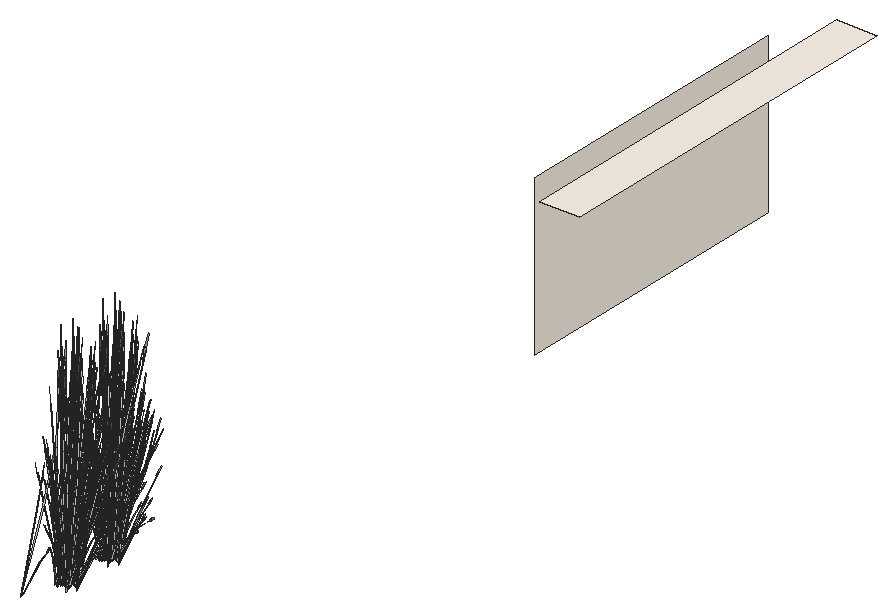
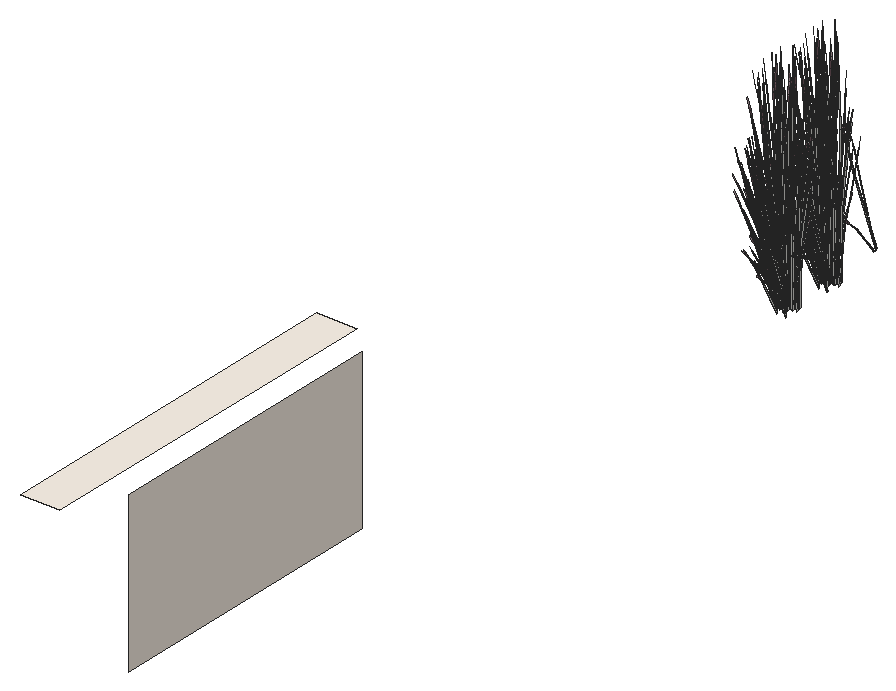
# SketchUp Ruby script. Lengths in inches.
U = 1.inch
M = Sketchup.active_model
def pt(a) = Geom::Point3d.new(a.map { |v| v * U })
def face(e, loops, mat)
  f = e.add_face(loops[0].map { |a| pt(a) })
  loops[1..].each { |l| e.add_face(l.map { |a| pt(a) }).erase! }
  f.material = f.back_material = mat if mat
  f
end
# faces: each face lists its corners as indices into pts; further lists are holes
def faces(e, pts, list, mat = nil) = list.each { |f| face(e, (f[0].is_a?(Array) ? f : [f]).map { |l| l.map { |i| pts[i] } }, mat) }
# xy, xz, yz: faces in a plane at the given z, y or x. An outline is a flat list of corners, or four numbers for a rectangle; further outlines are holes
def ring(l) = l.size == 4 ? [[l[0], l[1]], [l[2], l[1]], [l[2], l[3]], [l[0], l[3]]] : l.each_slice(2).to_a
def flat(e, list, mat, &to3) = list.each { |f| face(e, (f[0].is_a?(Array) ? f : [f]).map { |l| ring(l).map { |u, v| to3.(u, v) } }, mat) }
def xy(e, z, list, mat = nil) = flat(e, list, mat) { |x, y| [x, y, z] }
def xz(e, y, list, mat = nil) = flat(e, list, mat) { |x, z| [x, y, z] }
def yz(e, x, list, mat = nil) = flat(e, list, mat) { |y, z| [x, y, z] }
def lines(e, pts, list) = list.each { |a, b| e.add_line(pt(pts[a]), pt(pts[b])) }
# prism: a flat outline (further loops are holes) pulled along v
def prism(e, loops, v, mat = nil)
  f = face(e, loops, mat); d = Geom::Vector3d.new(v.map { |x| x * U })
  f.pushpull(f.normal.samedirection?(d) ? d.length : -d.length)
end
def box(e, o, s, mat = nil) = prism(e, [[o, [o[0] + s[0], o[1], o[2]], [o[0] + s[0], o[1] + s[1], o[2]], [o[0], o[1] + s[1], o[2]]]], [0, 0, s[2]], mat)
def at(x, y, z, deg = 0) = Geom::Transformation.translation(pt([x, y, z])) * Geom::Transformation.rotation(ORIGIN, Z_AXIS, deg.degrees)
def axes(o, x, y, z) = Geom::Transformation.new([*x, 0, *y, 0, *z, 0, *pt(o).to_a, 1])
def part(name) = M.definitions.add(name)
# library, detail: a bought-in or finely detailed component or shape, given as its bounding box
def library(name, o, s) = part(name).tap { |d| box(d.entities, o, s) }
def detail(e, o, s) = box(e.add_group.entities, o, s)
def put(e, d, t, mat = nil) = e.add_instance(d, t).tap { |i| i.material = mat if mat }
def group(e, t, mat = nil) = e.add_group.tap { |g| g.transformation = t; g.material = mat if mat }.entities
root = M.entities
M.materials.add("C01_Vanilla_Cream").color = [255, 246, 235]
M.materials.add("LightPink_Translucent").color = [144, 107, 117]
M.materials["LightPink_Translucent"].alpha = 0.75
c1 = part("blade")
p = [[2.15,0.21,22],[0,0.17,0],[0.09,0.45,0],[2.18,0.31,22],[2.29,0.31,22],[0.38,0.45,0],
  [2.48,0.24,33],[2.49,0.24,33],[2.48,0.22,33]]
faces(c1.entities,p,[[0,1,2,3],[4,5,2,3],[6,3,4,7],[8,0,3,6]])
c2 = part("seeds")
p = [[0.3,-0.1,1.38],[-0.01,-0.03,1.59],[-0.01,-0.03,0.03],[0.14,-0.07,-0.07],[0.29,-0.03,3],[0.15,0.01,3.11]]
faces(c2.entities,p,[[0,1,2,3],[1,0,4,5]],"LightPink_Translucent")
c3 = part("blade with seeds")
put(c3.entities,c1,at(0,0,0))
put(c3.entities,c2,axes([2.4,0.25,30.99],[1.5799,-0.05474,1.17369],[-0.12525,1.92788,0.29478],[-0.07173,-0.02425,1.56792]))
xy(root,690,[[360,288,369,372]],"C01_Vanilla_Cream")
yz(root,354,[[294,654,360,690]],"C01_Vanilla_Cream")
put(root,c3,axes([341.72,163.8,657.71],[-0.14896,0.31857,-0.29039],[-0.4346,-0.09292,0.3749],[0.03985,0.12826,0.71734]))
put(root,c3,axes([341.77,163.52,658.08],[0.23583,0.33684,-0.58257],[-0.48546,0.18772,0.0703],[0.05515,0.16275,0.8241]))
put(root,c3,axes([341.41,164.37,657.87],[0.06263,0.06671,1.43454],[0.50546,0.02621,-0.22687],[0.05083,0.14712,0.11505]))
put(root,c3,axes([343.01,173.53,656.125],[-0.14045,0.08385,1.17261],[-0.42064,-0.14676,-0.25218],[0.07797,-0.18252,0.50135]))
put(root,c3,axes([343.35,174.15,658.08],[0.01286,-0.38319,-0.58257],[0.54141,0.02574,0.0703],[0.05714,-0.16234,0.8241]))
put(root,c3,axes([344.11,173.55,657.87],[-0.00477,-0.08245,1.43454],[-0.40285,-0.23829,-0.22687],[0.06228,-0.14445,0.11505]))
put(root,c3,axes([342.41,173.54,657.71],[0.14896,-0.31857,-0.29039],[0.4346,0.09292,0.3749],[-0.03985,-0.12826,0.71734]))
put(root,c3,axes([342.74,173.96,657.18],[-0.092,0.14239,1.40529],[-0.38596,-0.29467,0.11363],[0.17411,-0.18366,0.60075]))
put(root,c3,axes([344,173.26,657.86],[-0.05018,0.03164,1.45454],[-0.49165,-0.10676,-0.13744],[-0.0178,-0.13809,0.2574]))
put(root,c3,axes([342.49,172.86,656.27],[0.06339,0.24157,0.94186],[-0.35163,-0.13379,0.69201],[0.03784,-0.12369,0.20745]))
put(root,c3,axes([343.24,174.02,657.84],[-0.35372,-0.27835,-0.41901],[0.37366,-0.24377,-0.32456],[0.05382,-0.14142,0.80174]))
put(root,c3,axes([342.47,173.61,657.88],[0.48688,0.1083,0.39362],[-0.16649,0.35605,0.32456],[-0.02926,-0.14002,0.8145]))
put(root,c3,axes([343.61,174.17,658.13],[-0.54305,-0.02053,-0.09971],[0.01484,-0.38862,-0.55346],[0.03772,-0.14967,0.84097]))
put(root,c3,axes([343.57,173.92,657.71],[0.33433,-0.21811,-0.29039],[0.31649,0.24905,0.3749],[0.04815,-0.12654,0.71734]))
put(root,c3,axes([342.6,173.58,657.88],[0.36409,-0.14079,0.05273],[0.17821,0.25674,0.41509],[-0.03516,-0.11317,0.63295]))
put(root,c3,axes([343.99,173.79,655.22],[-0.07396,-0.03263,1.44601],[-0.18997,-0.3646,-0.2209],[0.12815,-0.09894,0.2463]))
put(root,c3,axes([343.57,174.01,657.88],[0.35185,0.28265,0.39362],[-0.37366,0.24377,0.32456],[0.0649,-0.13261,0.8145]))
put(root,c3,axes([343.7,174.03,657.88],[0.40605,0.0193,0.05273],[-0.01113,0.29147,0.41509],[0.04249,-0.11165,0.63295]))
put(root,c3,axes([343.4,174.23,658.14],[-0.33433,0.21811,0.29039],[-0.31649,-0.24905,-0.3749],[0.04815,-0.12654,0.71734]))
put(root,c3,axes([343.99,174.82,658.08],[0.2581,-0.32687,-0.58257],[0.45228,0.2323,0.0703],[0.15411,-0.11843,0.8241]))
put(root,c3,axes([341.2,173.87,655.95],[-0.30893,-0.41511,0],[0.51685,-0.2315,-0.42318],[0.11772,-0.05273,1.34243]))
put(root,c3,axes([343.98,174.67,657.84],[-0.12693,-0.37826,-0.41901],[0.48071,-0.06617,-0.32456],[0.13776,-0.1016,0.80174]))
put(root,c3,axes([344.2,174.9375,658.13],[-0.45707,-0.22842,-0.09971],[0.26332,-0.3308,-0.55346],[0.12913,-0.11499,0.84097]))
put(root,c3,axes([341.62,173.8,655.65],[0.46245,-0.20713,-0.40713],[0.27641,0.37142,0],[0.10533,-0.04718,1.29153]))
put(root,c3,axes([344.36,174.52,656.125],[-0.17652,-0.01227,1.17261],[-0.18084,-0.32916,-0.25218],[0.21685,-0.09312,0.50135]))
put(root,c3,axes([345.33,174.84,657.86],[-0.06454,-0.00315,1.45454],[-0.268,-0.33712,-0.13744],[0.10763,-0.11085,0.2574]))
put(root,c3,axes([342.17,174.65,655.6875],[0.33282,-0.31137,-0.51129],[0.41344,0.28235,-0.13419],[0.13336,-0.07767,1.12859]))
put(root,c3,axes([344.57,173.91,656.27],[-0.16458,0.21088,0.94186],[-0.14146,-0.28332,0.69201],[0.13593,-0.07099,0.20745]))
put(root,c3,axes([344.33,174.71,657.71],[0.43011,-0.0592,-0.29039],[0.11357,0.33844,0.3749],[0.12326,-0.0909,0.71734]))
put(root,c3,axes([341.59,175.2,655.8125],[0.23974,-0.37328,-0.36686],[0.49814,0.17965,0.17656],[0,-0.08605,1.17788]))
put(root,c3,axes([341.81,175.01,656.1875],[-0.05758,-0.4727,-0.23858],[0.59969,-0.02858,-0.41002],[0.1056,-0.06296,1.3096]))
put(root,c3,axes([343.98,174.91,658.14],[-0.43011,0.0592,0.29039],[-0.11357,-0.33844,-0.3749],[0.12326,-0.0909,0.71734]))
put(root,c3,axes([341.73,173.97,655.66],[0.46099,0.1025,-0.25402],[-0.11607,0.36097,0.25402],[0.09293,-0.04163,1.13959]))
put(root,c3,axes([344.37,174.85,657.88],[0.33921,0.17422,0.05273],[-0.19749,0.2481,0.41509],[0.10876,-0.08021,0.63295]))
put(root,c3,axes([344.27,174.78,657.88],[0.12254,0.38127,0.39362],[-0.48071,0.06617,0.32456],[0.14168,-0.08967,0.8145]))
put(root,c3,axes([345.57,175.24,657.87],[0.06857,-0.0631,1.43454],[-0.08776,-0.38707,-0.22687],[0.17204,-0.07339,0.11505]))
put(root,c3,axes([341.88,175.38,656],[0.55674,0.20078,0.19733],[-0.26794,0.4172,0.41002],[0,-0.09617,1.31645]))
put(root,c3,axes([341.7,175.1,656.23],[-0.53657,0.02557,0.36686],[-0.04852,-0.4245,-0.17656],[0.09606,-0.04302,1.17788]))
put(root,c3,axes([344.22,175.83,658.13],[-0.24861,-0.37512,-0.09971],[0.44125,-0.18434,-0.55346],[0.18594,-0.04949,0.84097]))
put(root,c3,axes([344.2,175.51,657.84],[0.13386,-0.37682,-0.41901],[0.45895,0.12916,-0.32456],[0.18478,-0.03455,0.80174]))
put(root,c3,axes([343.47,173.97,655.95],[0.30893,-0.41511,0],[0.51685,0.2315,-0.42318],[0.11772,0.05273,1.34243]))
put(root,c3,axes([341.69,175.26,655.9375],[0.21483,0.46323,0.37519],[-0.61383,0.16108,0.14723],[0.0075,-0.08512,1.30262]))
put(root,c3,axes([344.6875,175.61,655.625],[-0.31825,0.04971,1.16098],[-0.05066,-0.39572,0.06645],[0.2229,-0.0599,0.66064]))
put(root,c3,axes([345.27,175.26,655.85],[-0.30634,-0.2649,-0.0532],[0.33551,-0.24272,-0.24121],[0.09507,-0.01709,0.7956]))
put(root,c3,axes([342.46,175.3,655.81],[0,-0.47933,0],[0.61786,0,0],[0,0,1.47154]))
put(root,c3,axes([343.21,174.1875,656.03],[-0.46245,-0.20713,0.40713],[0.27641,-0.37142,0],[0.10533,0.04718,1.29153]))
put(root,c3,axes([344.11,175.64,658.08],[0.43419,-0.18296,-0.58257],[0.24197,0.37661,0.0703],[0.20979,-0.04278,0.8241]))
put(root,c3,axes([342.17,174.99,655.9375],[-0.40969,0.37595,0.37519],[-0.48673,-0.33186,0.14723],[0.09877,-0.03752,1.30262]))
put(root,c3,axes([341.45,174.375,656.03],[-0.14274,0.41171,0.14467],[-0.52234,-0.11651,0.28771],[0.09023,-0.00201,1.31534]))
put(root,c3,axes([344.05,175.71,658.14],[-0.41064,-0.11557,0.29039],[0.11977,-0.33716,-0.3749],[0.16533,-0.03092,0.71734]))
put(root,c3,axes([341.24,174.71,655.31],[-0.48636,0.16585,1.05721],[-0.1548,-0.47588,0.41079],[0.29865,0.00792,1.20246]))
put(root,c3,axes([342.54,174.83,656.15],[0.09532,-0.36971,0.11873],[0.46572,0.06418,-0.33905],[0.08476,0.03796,1.0393]))
put(root,c3,axes([345.04,175.35,655.22],[-0.02582,-0.06289,1.44601],[0.17911,-0.36789,-0.2209],[0.18067,-0.00529,0.2463]))
put(root,c3,axes([342.35,174.93,656.23],[-0.29683,-0.34771,0.36686],[0.44961,-0.24485,-0.17656],[0.09606,0.04302,1.17788]))
put(root,c3,axes([342.5,174.95,656.1875],[0.49889,-0.27503,-0.23858],[0.33175,0.38862,-0.41002],[0.12309,0.03947,1.3096]))
put(root,c3,axes([344.48,175.68,657.71],[0.41064,0.11557,-0.29039],[-0.11977,0.33716,0.3749],[0.16533,-0.03092,0.71734]))
put(root,c3,axes([343.75,174.22,655.65],[0.46245,0.20713,-0.40713],[-0.27641,0.37142,0],[0.10533,0.04718,1.29153]))
put(root,c3,axes([342.88,175.4,655.81],[0.55282,0,0],[0,0.42888,0],[0,0,1.46294]))
put(root,c3,axes([343.03,174.4,656.03],[-0.53096,0.10995,0.14467],[-0.13111,-0.40919,0.28771],[0.04735,0.05962,1.31534]))
put(root,c3,axes([343.36,175.26,657.18],[-0.20495,0.00938,1.40529],[0.13596,-0.40664,0.11363],[0.29207,0.02515,0.60075]))
put(root,c3,axes([343.625,174.375,655.66],[0.11607,0.36097,-0.25402],[-0.46099,0.1025,0.25402],[0.09293,0.04163,1.13959]))
put(root,c3,axes([344.42,175.82,657.88],[0.18148,0.28246,0.05273],[-0.33093,0.13825,0.41509],[0.14588,-0.02728,0.63295]))
put(root,c3,axes([342.7,175.18,655.95],[-0.62452,-0.08728,0.40343],[0.1271,-0.49295,0.15831],[0.09127,0.0476,1.40067]))
put(root,c3,axes([344.39,175.72,657.88],[-0.1396,0.37772,0.39362],[-0.45895,-0.12916,0.32456],[0.18049,-0.0227,0.8145]))
put(root,c3,axes([342.2,176.4,655.81],[-0.16122,-0.35715,0],[0.46037,-0.12507,0],[0,0,1.26584]))
put(root,c3,axes([342.8,176.35,655.79],[0.51876,-0.14056,-0.15742],[0.18228,0.40489,0.00007],[0.05726,-0.01554,1.42596]))
put(root,c3,axes([342.87,175.59,655.82],[0.34492,0.26758,0],[-0.34492,0.26758,0],[0,0,1.38798]))
put(root,c3,axes([343.8,175.47,656.03],[-0.38822,-0.30175,0.14467],[0.39123,-0.29268,0.28771],[-0.04288,0.06162,1.31534]))
put(root,c3,axes([343.08,175.01,655.6875],[0.514,0.06792,-0.51129],[-0.10846,0.41895,-0.13419],[0.15339,0.05076,1.12859]))
put(root,c3,axes([345.35,175.75,656.27],[-0.30529,0.06839,0.94186],[0.1437,-0.28265,0.69201],[0.16196,0.01934,0.20745]))
put(root,c3,axes([342.86,175.27,656.23],[0.23974,-0.37328,0.36686],[0.49814,0.17965,-0.17656],[0,0.08605,1.17788]))
put(root,c3,axes([345.21,176.94,657.86],[-0.04468,-0.03627,1.45454],[0.09773,-0.38875,-0.13744],[0.17599,-0.02484,0.2574]))
put(root,c3,axes([342.77,175.49,655.88],[0,0.4791,-0.04622],[-0.61786,0,0],[0,0.01506,1.47081]))
put(root,c3,axes([342.8125,175.15,655.8125],[0.29683,0.34771,-0.36686],[-0.44961,0.24485,0.17656],[0.09606,0.04302,1.17788]))
put(root,c3,axes([344.82,176.62,657.22],[-0.09457,-0.34824,-0.02863],[0.44699,-0.08006,-0.12982],[0.09334,0.02208,0.42819]))
put(root,c3,axes([343.66,176.61,658.13],[0.02646,-0.4213,-0.09971],[0.50094,0.01152,-0.55346],[0.19293,0.02926,0.84097]))
put(root,c3,axes([344.12,175.48,656.03],[0,-0.41426,0.40713],[0.55282,0,0],[0,0.09435,1.29153]))
put(root,c3,axes([343.07,175.36,656.15],[0.46037,-0.12081,0.11873],[0.16122,0.34498,-0.33905],[0,0.07592,1.0393]))
put(root,c3,axes([343.59,176.44,658.14],[-0.28114,-0.25937,0.29039],[0.32102,-0.24553,-0.3749],[0.16311,0.03736,0.71734]))
put(root,c3,axes([344.78,176.2,656.125],[-0.119,-0.10189,1.17261],[0.15483,-0.33705,-0.25218],[0.24077,0.04566,0.50135]))
put(root,c3,axes([342.65,176.57,655.81],[0.49814,0.18599,0],[-0.23974,0.38645,0],[0,0,1.43462]))
put(root,c3,axes([344.1,176.35,657.87],[0.106,-0.00701,1.43454],[0.29074,-0.32184,-0.22687],[0.18854,0.04248,0.11505]))
put(root,c3,axes([343.6875,176.4,658.08],[0.49394,0.00997,-0.58257],[-0.03317,0.42002,0.0703],[0.20925,0.04433,0.8241]))
put(root,c3,axes([342.47,176.41,655.88],[0.21483,0.47591,-0.0493],[-0.61383,0.16676,0],[0.0075,0.01662,1.41182]))
put(root,c3,axes([344.49,175.55,655.95],[0.61786,0,0],[0,0.463,-0.42318],[0,0.10545,1.34243]))
put(root,c3,axes([344.25,175.79,655.8],[-0.61756,-0.00331,-0.04081],[0,-0.463,0.40953],[-0.01941,0.1054,1.29849]))
put(root,c3,axes([342.91,175.39,656.1875],[0.55647,0.19766,-0.23858],[-0.26794,0.4172,-0.41002],[0.01749,0.10243,1.3096]))
put(root,c3,axes([343.98,176.58,657.71],[0.28114,0.25937,-0.29039],[-0.32102,0.24553,0.3749],[0.16311,0.03736,0.71734]))
put(root,c3,axes([344.12,175.86,655.66],[-0.34492,0.25847,-0.25402],[-0.34492,-0.25847,0.25402],[0,0.08325,1.13959]))
put(root,c3,axes([343.84,176.68,657.88],[-0.02488,0.31501,0.05273],[-0.3757,-0.00864,0.41509],[0.14392,0.03296,0.63295]))
put(root,c3,axes([342.85,175.7,655.8125],[-0.23974,0.37328,-0.36686],[-0.49814,-0.17965,0.17656],[0,0.08605,1.17788]))
put(root,c3,axes([343.875,176.58,657.88],[-0.36434,0.27297,0.39362],[-0.31422,-0.28988,0.32456],[0.17094,0.05035,0.8145]))
put(root,c3,axes([342.72,176.89,658.14],[-0.07631,-0.33368,0.29039],[0.43626,-0.08811,-0.3749],[0.11718,0.09562,0.71734]))
put(root,c3,axes([344.36,175.87,655.65],[0,0.41426,-0.40713],[-0.55282,0,0],[0,0.09435,1.29153]))
put(root,c3,axes([342.97,175.91,657.18],[-0.18354,-0.07137,1.40529],[0.37983,-0.29943,0.11363],[0.23673,0.13508,0.60075]))
put(root,c3,axes([343.01,174.97,657.67],[-0.42697,-0.21524,1.13392],[0.45084,-0.33512,0.48925],[0.13776,0.20196,1.09604]))
put(root,c3,axes([343.65,176.73,656.27],[-0.27821,-0.11912,0.94186],[0.35924,-0.12103,0.69201],[0.09689,0.10252,0.20745]))
put(root,c3,axes([342.68,177.07,658.13],[0.29444,-0.35459,-0.09971],[0.4264,0.20428,-0.55346],[0.14822,0.10018,0.84097]))
put(root,c3,axes([342.29,177.36,657.86],[0.00146,-0.05015,1.45454],[0.42344,-0.22127,-0.13744],[0.14708,0.07898,0.2574]))
put(root,c3,axes([343.73,177.17,655.22],[0.036,-0.05981,1.44601],[0.45322,-0.17614,-0.2209],[0.1374,0.09116,0.2463]))
put(root,c3,axes([343.13,175.81,655.72],[0.18118,0.37929,-0.56754],[-0.52191,0.1366,-0.14895],[0.02003,0.12844,1.25274]))
put(root,c3,axes([343.03,176.89,657.84],[0.48758,-0.09847,-0.41901],[0.08529,0.37293,-0.32456],[0.13096,0.10687,0.80174]))
put(root,c3,axes([341.67,176.95,658.14],[0.14896,-0.31857,0.29039],[0.4346,0.09292,-0.3749],[0.03985,0.12826,0.71734]))
put(root,c3,axes([343.7,177.27,656.1875],[-0.31686,-0.01299,0.86149],[0.20925,-0.27594,0.47565],[0.12517,0.09804,0.67577]))
put(root,c3,axes([342.79,177.2,657.88],[-0.22457,0.26316,0.05273],[-0.3198,-0.15321,0.41509],[0.10339,0.08437,0.63295]))
put(root,c3,axes([342.26,178.08,658.63],[0.34145,-0.23766,-0.0532],[0.31287,0.26029,-0.24121],[0.02203,0.07375,0.7956]))
put(root,c3,axes([342.88,177.12,657.88],[-0.49145,0.09507,0.39362],[-0.08529,-0.37293,0.32456],[0.11558,0.10991,0.8145]))
put(root,c3,axes([342.66,176.6,656.125],[0.00872,-0.13732,1.17261],[0.41669,-0.15339,-0.25218],[0.12863,0.16436,0.50135]))
put(root,c3,axes([341.53,177.08,658.13],[0.48353,-0.19287,-0.09971],[0.23761,0.34232,-0.55346],[0.0638,0.14425,0.84097]))
put(root,c3,axes([341.61,177.15,655.22],[0.07997,-0.02254,1.44601],[0.48102,0.12407,-0.2209],[0.01407,0.13984,0.2463]))
put(root,c3,axes([341.94,177.0625,657.84],[0.48573,0.10385,-0.41901],[-0.16649,0.35605,-0.32456],[0.04454,0.14335,0.80174]))
put(root,c3,axes([342.22,176.33,657.18],[-0.11295,-0.13301,1.40529],[0.52192,-0.11198,0.11363],[0.11796,0.20881,0.60075]))
put(root,c3,axes([341.72,177.28,657.71],[-0.14896,0.31857,-0.29039],[-0.4346,-0.09292,0.3749],[0.03985,0.12826,0.71734]))
put(root,c3,axes([341.77,177,658.08],[0.23583,0.33684,-0.58257],[-0.48546,0.18772,0.0703],[0.05515,0.16275,0.8241]))
put(root,c3,axes([341.41,177.85,657.87],[0.06263,0.06671,1.43454],[0.50546,0.02621,-0.22687],[0.05083,0.14712,0.11505]))
put(root,c3,axes([343.01,185.39,656.125],[-0.14045,0.08385,1.17261],[-0.42064,-0.14676,-0.25218],[0.07797,-0.18252,0.50135]))
put(root,c3,axes([343.35,186.01,658.08],[0.01286,-0.38319,-0.58257],[0.54141,0.02574,0.0703],[0.05714,-0.16234,0.8241]))
put(root,c3,axes([344.11,185.42,657.87],[-0.00477,-0.08245,1.43454],[-0.40285,-0.23829,-0.22687],[0.06228,-0.14445,0.11505]))
put(root,c3,axes([342.41,185.4,657.71],[0.14896,-0.31857,-0.29039],[0.4346,0.09292,0.3749],[-0.03985,-0.12826,0.71734]))
put(root,c3,axes([342.74,185.82,657.18],[-0.092,0.14239,1.40529],[-0.38596,-0.29467,0.11363],[0.17411,-0.18366,0.60075]))
put(root,c3,axes([344,185.12,657.86],[-0.05018,0.03164,1.45454],[-0.49165,-0.10676,-0.13744],[-0.0178,-0.13809,0.2574]))
put(root,c3,axes([342.49,184.72,656.27],[0.06339,0.24157,0.94186],[-0.35163,-0.13379,0.69201],[0.03784,-0.12369,0.20745]))
put(root,c3,axes([343.24,185.89,657.84],[-0.35372,-0.27835,-0.41901],[0.37366,-0.24377,-0.32456],[0.05382,-0.14142,0.80174]))
put(root,c3,axes([342.47,185.47,657.88],[0.48688,0.1083,0.39362],[-0.16649,0.35605,0.32456],[-0.02926,-0.14002,0.8145]))
put(root,c3,axes([343.61,186.03,658.13],[-0.54305,-0.02053,-0.09971],[0.01484,-0.38862,-0.55346],[0.03772,-0.14967,0.84097]))
put(root,c3,axes([343.57,185.78,657.71],[0.33433,-0.21811,-0.29039],[0.31649,0.24905,0.3749],[0.04815,-0.12654,0.71734]))
put(root,c3,axes([342.6,185.44,657.88],[0.36409,-0.14079,0.05273],[0.17821,0.25674,0.41509],[-0.03516,-0.11317,0.63295]))
put(root,c3,axes([343.99,185.65,655.22],[-0.07396,-0.03263,1.44601],[-0.18997,-0.3646,-0.2209],[0.12815,-0.09894,0.2463]))
put(root,c3,axes([343.57,185.87,657.88],[0.35185,0.28265,0.39362],[-0.37366,0.24377,0.32456],[0.0649,-0.13261,0.8145]))
put(root,c3,axes([343.7,185.89,657.88],[0.40605,0.0193,0.05273],[-0.01113,0.29147,0.41509],[0.04249,-0.11165,0.63295]))
put(root,c3,axes([343.4,186.09,658.14],[-0.33433,0.21811,0.29039],[-0.31649,-0.24905,-0.3749],[0.04815,-0.12654,0.71734]))
put(root,c3,axes([343.99,186.68,658.08],[0.2581,-0.32687,-0.58257],[0.45228,0.2323,0.0703],[0.15411,-0.11843,0.8241]))
put(root,c3,axes([341.2,185.73,655.95],[-0.30893,-0.41511,0],[0.51685,-0.2315,-0.42318],[0.11772,-0.05273,1.34243]))
put(root,c3,axes([343.98,186.53,657.84],[-0.12693,-0.37826,-0.41901],[0.48071,-0.06617,-0.32456],[0.13776,-0.1016,0.80174]))
put(root,c3,axes([344.2,186.8,658.13],[-0.45707,-0.22842,-0.09971],[0.26332,-0.3308,-0.55346],[0.12913,-0.11499,0.84097]))
put(root,c3,axes([341.62,185.66,655.65],[0.46245,-0.20713,-0.40713],[0.27641,0.37142,0],[0.10533,-0.04718,1.29153]))
put(root,c3,axes([344.36,186.38,656.125],[-0.17652,-0.01227,1.17261],[-0.18084,-0.32916,-0.25218],[0.21685,-0.09312,0.50135]))
put(root,c3,axes([345.33,186.7,657.86],[-0.06454,-0.00315,1.45454],[-0.268,-0.33712,-0.13744],[0.10763,-0.11085,0.2574]))
put(root,c3,axes([342.17,186.51,655.6875],[0.33282,-0.31137,-0.51129],[0.41344,0.28235,-0.13419],[0.13336,-0.07767,1.12859]))
put(root,c3,axes([344.57,185.77,656.27],[-0.16458,0.21088,0.94186],[-0.14146,-0.28332,0.69201],[0.13593,-0.07099,0.20745]))
put(root,c3,axes([344.33,186.57,657.71],[0.43011,-0.0592,-0.29039],[0.11357,0.33844,0.3749],[0.12326,-0.0909,0.71734]))
put(root,c3,axes([341.59,187.06,655.8125],[0.23974,-0.37328,-0.36686],[0.49814,0.17965,0.17656],[0,-0.08605,1.17788]))
put(root,c3,axes([341.81,186.875,656.1875],[-0.05758,-0.4727,-0.23858],[0.59969,-0.02858,-0.41002],[0.1056,-0.06296,1.3096]))
put(root,c3,axes([343.98,186.77,658.14],[-0.43011,0.0592,0.29039],[-0.11357,-0.33844,-0.3749],[0.12326,-0.0909,0.71734]))
put(root,c3,axes([341.73,185.83,655.66],[0.46099,0.1025,-0.25402],[-0.11607,0.36097,0.25402],[0.09293,-0.04163,1.13959]))
put(root,c3,axes([344.37,186.71,657.88],[0.33921,0.17422,0.05273],[-0.19749,0.2481,0.41509],[0.10876,-0.08021,0.63295]))
put(root,c3,axes([344.27,186.64,657.88],[0.12254,0.38127,0.39362],[-0.48071,0.06617,0.32456],[0.14168,-0.08967,0.8145]))
put(root,c3,axes([345.57,187.1,657.87],[0.06857,-0.0631,1.43454],[-0.08776,-0.38707,-0.22687],[0.17204,-0.07339,0.11505]))
put(root,c3,axes([341.88,187.24,656],[0.55674,0.20078,0.19733],[-0.26794,0.4172,0.41002],[0,-0.09617,1.31645]))
put(root,c3,axes([341.7,186.96,656.23],[-0.53657,0.02557,0.36686],[-0.04852,-0.4245,-0.17656],[0.09606,-0.04302,1.17788]))
put(root,c3,axes([344.22,187.6875,658.13],[-0.24861,-0.37512,-0.09971],[0.44125,-0.18434,-0.55346],[0.18594,-0.04949,0.84097]))
put(root,c3,axes([344.2,187.37,657.84],[0.13386,-0.37682,-0.41901],[0.45895,0.12916,-0.32456],[0.18478,-0.03455,0.80174]))
put(root,c3,axes([343.47,185.83,655.95],[0.30893,-0.41511,0],[0.51685,0.2315,-0.42318],[0.11772,0.05273,1.34243]))
put(root,c3,axes([341.69,187.12,655.9375],[0.21483,0.46323,0.37519],[-0.61383,0.16108,0.14723],[0.0075,-0.08512,1.30262]))
put(root,c3,axes([344.6875,187.47,655.625],[-0.31825,0.04971,1.16098],[-0.05066,-0.39572,0.06645],[0.2229,-0.0599,0.66064]))
put(root,c3,axes([345.27,187.12,655.85],[-0.30634,-0.2649,-0.0532],[0.33551,-0.24272,-0.24121],[0.09507,-0.01709,0.7956]))
put(root,c3,axes([342.46,187.16,655.81],[0,-0.47933,0],[0.61786,0,0],[0,0,1.47154]))
put(root,c3,axes([343.21,186.05,656.03],[-0.46245,-0.20713,0.40713],[0.27641,-0.37142,0],[0.10533,0.04718,1.29153]))
put(root,c3,axes([344.11,187.5,658.08],[0.43419,-0.18296,-0.58257],[0.24197,0.37661,0.0703],[0.20979,-0.04278,0.8241]))
put(root,c3,axes([342.17,186.86,655.9375],[-0.40969,0.37595,0.37519],[-0.48673,-0.33186,0.14723],[0.09877,-0.03752,1.30262]))
put(root,c3,axes([341.45,186.24,656.03],[-0.14274,0.41171,0.14467],[-0.52234,-0.11651,0.28771],[0.09023,-0.00201,1.31534]))
put(root,c3,axes([344.05,187.58,658.14],[-0.41064,-0.11557,0.29039],[0.11977,-0.33716,-0.3749],[0.16533,-0.03092,0.71734]))
put(root,c3,axes([341.24,186.57,655.31],[-0.48636,0.16585,1.05721],[-0.1548,-0.47588,0.41079],[0.29865,0.00792,1.20246]))
put(root,c3,axes([342.54,186.69,656.15],[0.09532,-0.36971,0.11873],[0.46572,0.06418,-0.33905],[0.08476,0.03796,1.0393]))
put(root,c3,axes([345.04,187.21,655.22],[-0.02582,-0.06289,1.44601],[0.17911,-0.36789,-0.2209],[0.18067,-0.00529,0.2463]))
put(root,c3,axes([342.35,186.79,656.23],[-0.29683,-0.34771,0.36686],[0.44961,-0.24485,-0.17656],[0.09606,0.04302,1.17788]))
put(root,c3,axes([342.5,186.8125,656.1875],[0.49889,-0.27503,-0.23858],[0.33175,0.38862,-0.41002],[0.12309,0.03947,1.3096]))
put(root,c3,axes([344.48,187.54,657.71],[0.41064,0.11557,-0.29039],[-0.11977,0.33716,0.3749],[0.16533,-0.03092,0.71734]))
put(root,c3,axes([343.75,186.08,655.65],[0.46245,0.20713,-0.40713],[-0.27641,0.37142,0],[0.10533,0.04718,1.29153]))
put(root,c3,axes([342.88,187.26,655.81],[0.55282,0,0],[0,0.42888,0],[0,0,1.46294]))
put(root,c3,axes([343.03,186.26,656.03],[-0.53096,0.10995,0.14467],[-0.13111,-0.40919,0.28771],[0.04735,0.05962,1.31534]))
put(root,c3,axes([343.36,187.12,657.18],[-0.20495,0.00938,1.40529],[0.13596,-0.40664,0.11363],[0.29207,0.02515,0.60075]))
put(root,c3,axes([343.625,186.24,655.66],[0.11607,0.36097,-0.25402],[-0.46099,0.1025,0.25402],[0.09293,0.04163,1.13959]))
put(root,c3,axes([344.42,187.68,657.88],[0.18148,0.28246,0.05273],[-0.33093,0.13825,0.41509],[0.14588,-0.02728,0.63295]))
put(root,c3,axes([342.7,187.05,655.95],[-0.62452,-0.08728,0.40343],[0.1271,-0.49295,0.15831],[0.09127,0.0476,1.40067]))
put(root,c3,axes([344.39,187.58,657.88],[-0.1396,0.37772,0.39362],[-0.45895,-0.12916,0.32456],[0.18049,-0.0227,0.8145]))
put(root,c3,axes([342.2,188.26,655.81],[-0.16122,-0.35715,0],[0.46037,-0.12507,0],[0,0,1.26584]))
put(root,c3,axes([342.8,188.21,655.79],[0.51876,-0.14056,-0.15742],[0.18228,0.40489,0.00007],[0.05726,-0.01554,1.42596]))
put(root,c3,axes([342.87,187.45,655.82],[0.34492,0.26758,0],[-0.34492,0.26758,0],[0,0,1.38798]))
put(root,c3,axes([343.8,187.33,656.03],[-0.38822,-0.30175,0.14467],[0.39123,-0.29268,0.28771],[-0.04288,0.06162,1.31534]))
put(root,c3,axes([343.08,186.875,655.6875],[0.514,0.06792,-0.51129],[-0.10846,0.41895,-0.13419],[0.15339,0.05076,1.12859]))
put(root,c3,axes([345.35,187.61,656.27],[-0.30529,0.06839,0.94186],[0.1437,-0.28265,0.69201],[0.16196,0.01934,0.20745]))
put(root,c3,axes([342.86,187.14,656.23],[0.23974,-0.37328,0.36686],[0.49814,0.17965,-0.17656],[0,0.08605,1.17788]))
put(root,c3,axes([345.21,188.8,657.86],[-0.04468,-0.03627,1.45454],[0.09773,-0.38875,-0.13744],[0.17599,-0.02484,0.2574]))
put(root,c3,axes([342.77,187.35,655.88],[0,0.4791,-0.04622],[-0.61786,0,0],[0,0.01506,1.47081]))
put(root,c3,axes([342.8125,187.01,655.8125],[0.29683,0.34771,-0.36686],[-0.44961,0.24485,0.17656],[0.09606,0.04302,1.17788]))
put(root,c3,axes([344.82,188.48,657.22],[-0.09457,-0.34824,-0.02863],[0.44699,-0.08006,-0.12982],[0.09334,0.02208,0.42819]))
put(root,c3,axes([343.66,188.47,658.13],[0.02646,-0.4213,-0.09971],[0.50094,0.01152,-0.55346],[0.19293,0.02926,0.84097]))
put(root,c3,axes([344.12,187.34,656.03],[0,-0.41426,0.40713],[0.55282,0,0],[0,0.09435,1.29153]))
put(root,c3,axes([343.07,187.22,656.15],[0.46037,-0.12081,0.11873],[0.16122,0.34498,-0.33905],[0,0.07592,1.0393]))
put(root,c3,axes([343.59,188.3,658.14],[-0.28114,-0.25937,0.29039],[0.32102,-0.24553,-0.3749],[0.16311,0.03736,0.71734]))
put(root,c3,axes([344.78,188.0625,656.125],[-0.119,-0.10189,1.17261],[0.15483,-0.33705,-0.25218],[0.24077,0.04566,0.50135]))
put(root,c3,axes([342.65,188.43,655.81],[0.49814,0.18599,0],[-0.23974,0.38645,0],[0,0,1.43462]))
put(root,c3,axes([344.1,188.22,657.87],[0.106,-0.00701,1.43454],[0.29074,-0.32184,-0.22687],[0.18854,0.04248,0.11505]))
put(root,c3,axes([343.6875,188.27,658.08],[0.49394,0.00997,-0.58257],[-0.03317,0.42002,0.0703],[0.20925,0.04433,0.8241]))
put(root,c3,axes([342.47,188.28,655.88],[0.21483,0.47591,-0.0493],[-0.61383,0.16676,0],[0.0075,0.01662,1.41182]))
put(root,c3,axes([344.49,187.41,655.95],[0.61786,0,0],[0,0.463,-0.42318],[0,0.10545,1.34243]))
put(root,c3,axes([344.25,187.65,655.8],[-0.61756,-0.00331,-0.04081],[0,-0.463,0.40953],[-0.01941,0.1054,1.29849]))
put(root,c3,axes([342.91,187.25,656.1875],[0.55647,0.19766,-0.23858],[-0.26794,0.4172,-0.41002],[0.01749,0.10243,1.3096]))
put(root,c3,axes([343.98,188.4375,657.71],[0.28114,0.25937,-0.29039],[-0.32102,0.24553,0.3749],[0.16311,0.03736,0.71734]))
put(root,c3,axes([344.12,187.72,655.66],[-0.34492,0.25847,-0.25402],[-0.34492,-0.25847,0.25402],[0,0.08325,1.13959]))
put(root,c3,axes([343.84,188.54,657.88],[-0.02488,0.31501,0.05273],[-0.3757,-0.00864,0.41509],[0.14392,0.03296,0.63295]))
put(root,c3,axes([342.85,187.56,655.8125],[-0.23974,0.37328,-0.36686],[-0.49814,-0.17965,0.17656],[0,0.08605,1.17788]))
put(root,c3,axes([343.875,188.4375,657.88],[-0.36434,0.27297,0.39362],[-0.31422,-0.28988,0.32456],[0.17094,0.05035,0.8145]))
put(root,c3,axes([342.72,188.75,658.14],[-0.07631,-0.33368,0.29039],[0.43626,-0.08811,-0.3749],[0.11718,0.09562,0.71734]))
put(root,c3,axes([344.36,187.73,655.65],[0,0.41426,-0.40713],[-0.55282,0,0],[0,0.09435,1.29153]))
put(root,c3,axes([342.97,187.77,657.18],[-0.18354,-0.07137,1.40529],[0.37983,-0.29943,0.11363],[0.23673,0.13508,0.60075]))
put(root,c3,axes([343.01,186.83,657.67],[-0.42697,-0.21524,1.13392],[0.45084,-0.33512,0.48925],[0.13776,0.20196,1.09604]))
put(root,c3,axes([343.65,188.59,656.27],[-0.27821,-0.11912,0.94186],[0.35924,-0.12103,0.69201],[0.09689,0.10252,0.20745]))
put(root,c3,axes([342.68,188.93,658.13],[0.29444,-0.35459,-0.09971],[0.4264,0.20428,-0.55346],[0.14822,0.10018,0.84097]))
put(root,c3,axes([342.29,189.22,657.86],[0.00146,-0.05015,1.45454],[0.42344,-0.22127,-0.13744],[0.14708,0.07898,0.2574]))
put(root,c3,axes([343.73,189.03,655.22],[0.036,-0.05981,1.44601],[0.45322,-0.17614,-0.2209],[0.1374,0.09116,0.2463]))
put(root,c3,axes([343.13,187.67,655.72],[0.18118,0.37929,-0.56754],[-0.52191,0.1366,-0.14895],[0.02003,0.12844,1.25274]))
put(root,c3,axes([343.03,188.75,657.84],[0.48758,-0.09847,-0.41901],[0.08529,0.37293,-0.32456],[0.13096,0.10687,0.80174]))
put(root,c3,axes([341.67,188.81,658.14],[0.14896,-0.31857,0.29039],[0.4346,0.09292,-0.3749],[0.03985,0.12826,0.71734]))
put(root,c3,axes([343.7,189.13,656.1875],[-0.31686,-0.01299,0.86149],[0.20925,-0.27594,0.47565],[0.12517,0.09804,0.67577]))
put(root,c3,axes([342.79,189.06,657.88],[-0.22457,0.26316,0.05273],[-0.3198,-0.15321,0.41509],[0.10339,0.08437,0.63295]))
put(root,c3,axes([342.26,189.94,658.63],[0.34145,-0.23766,-0.0532],[0.31287,0.26029,-0.24121],[0.02203,0.07375,0.7956]))
put(root,c3,axes([342.88,188.98,657.88],[-0.49145,0.09507,0.39362],[-0.08529,-0.37293,0.32456],[0.11558,0.10991,0.8145]))
put(root,c3,axes([342.66,188.46,656.125],[0.00872,-0.13732,1.17261],[0.41669,-0.15339,-0.25218],[0.12863,0.16436,0.50135]))
put(root,c3,axes([341.53,188.94,658.13],[0.48353,-0.19287,-0.09971],[0.23761,0.34232,-0.55346],[0.0638,0.14425,0.84097]))
put(root,c3,axes([341.61,189.02,655.22],[0.07997,-0.02254,1.44601],[0.48102,0.12407,-0.2209],[0.01407,0.13984,0.2463]))
put(root,c3,axes([341.94,188.92,657.84],[0.48573,0.10385,-0.41901],[-0.16649,0.35605,-0.32456],[0.04454,0.14335,0.80174]))
put(root,c3,axes([342.22,188.1875,657.18],[-0.11295,-0.13301,1.40529],[0.52192,-0.11198,0.11363],[0.11796,0.20881,0.60075]))
put(root,c3,axes([341.72,189.14,657.71],[-0.14896,0.31857,-0.29039],[-0.4346,-0.09292,0.3749],[0.03985,0.12826,0.71734]))
put(root,c3,axes([341.77,188.86,658.08],[0.23583,0.33684,-0.58257],[-0.48546,0.18772,0.0703],[0.05515,0.16275,0.8241]))
put(root,c3,axes([341.41,189.71,657.87],[0.06263,0.06671,1.43454],[0.50546,0.02621,-0.22687],[0.05083,0.14712,0.11505]))
